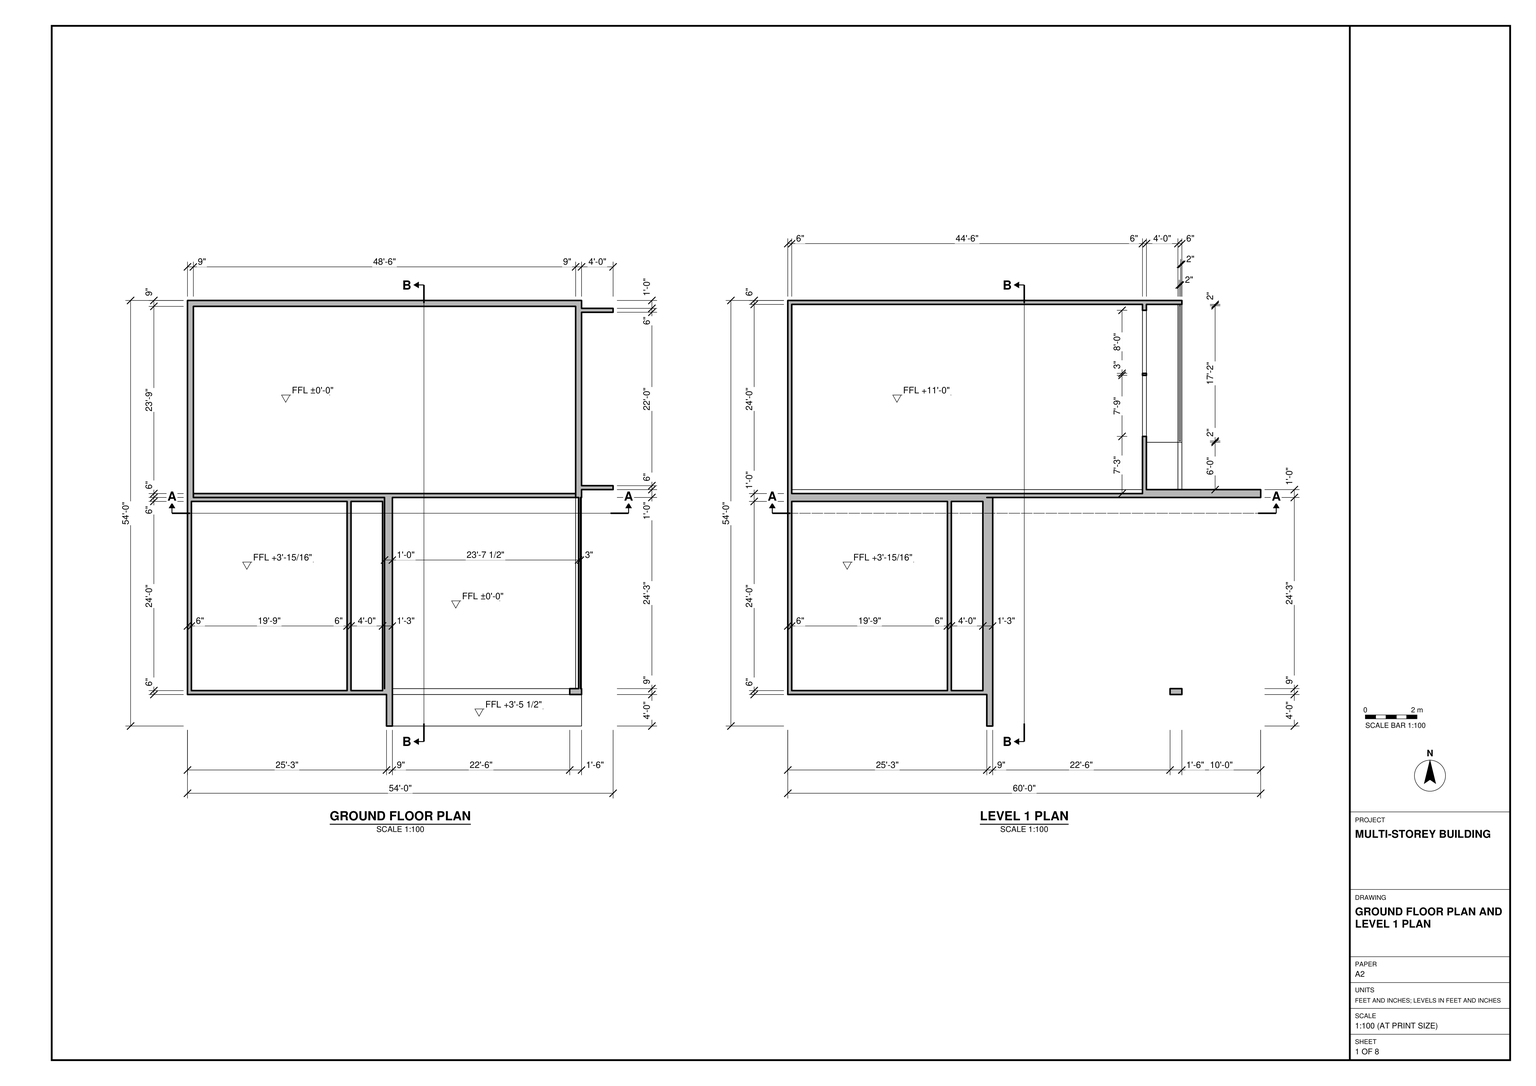
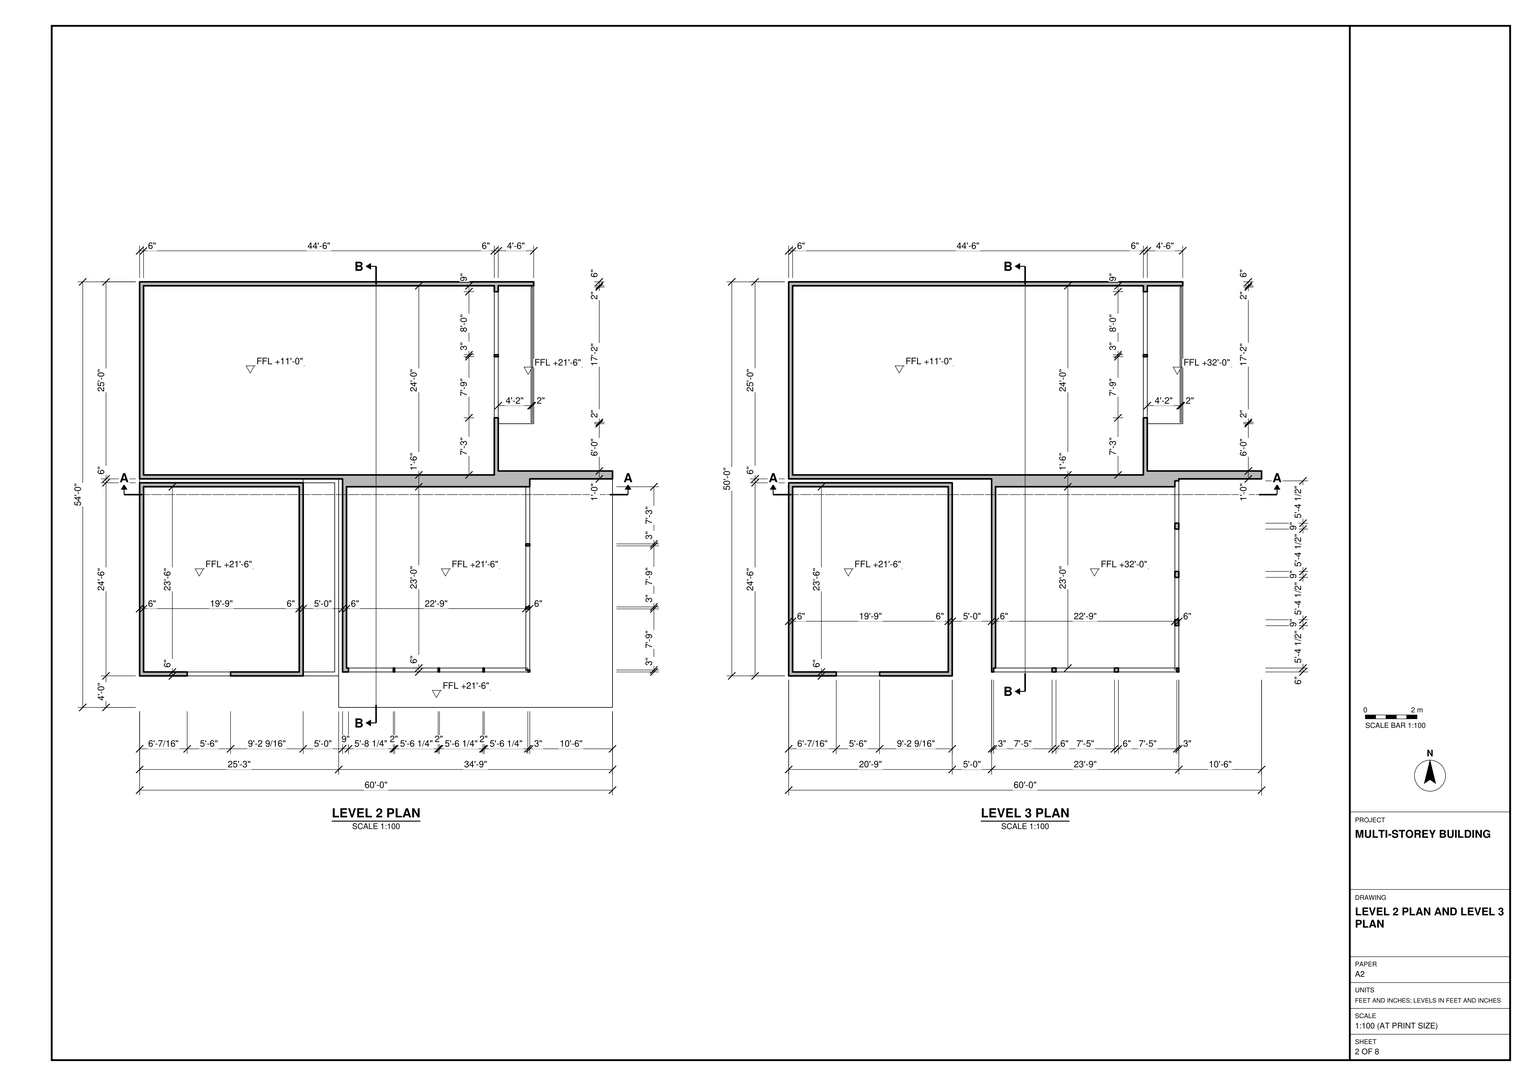
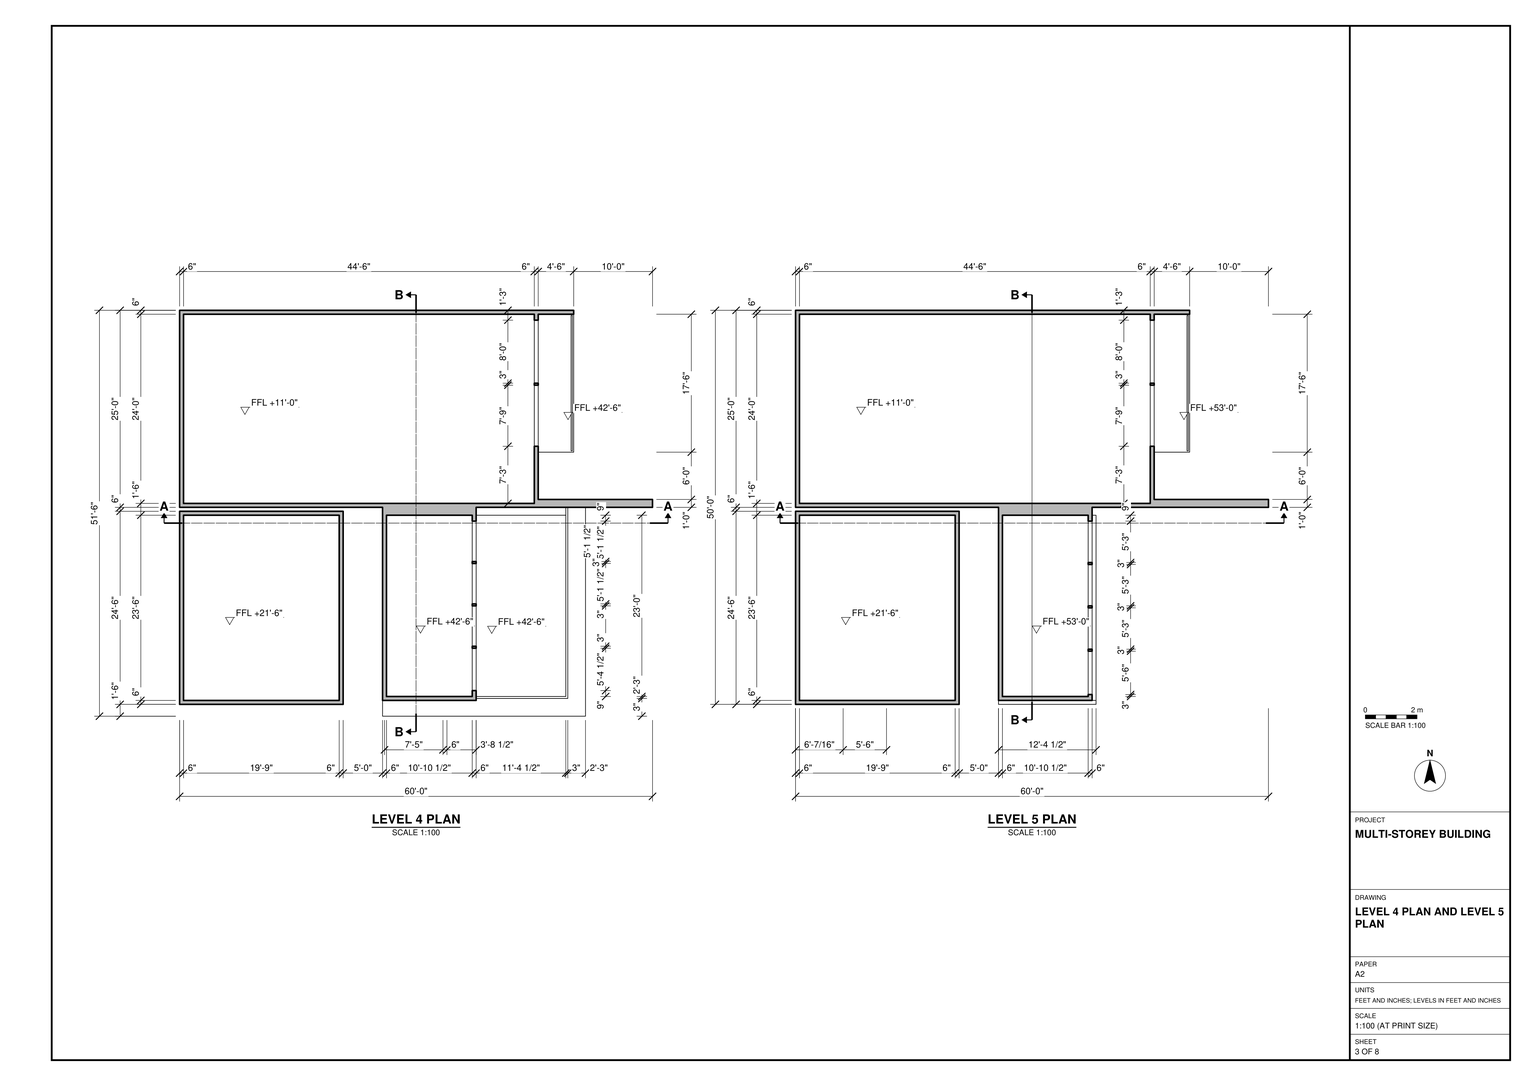
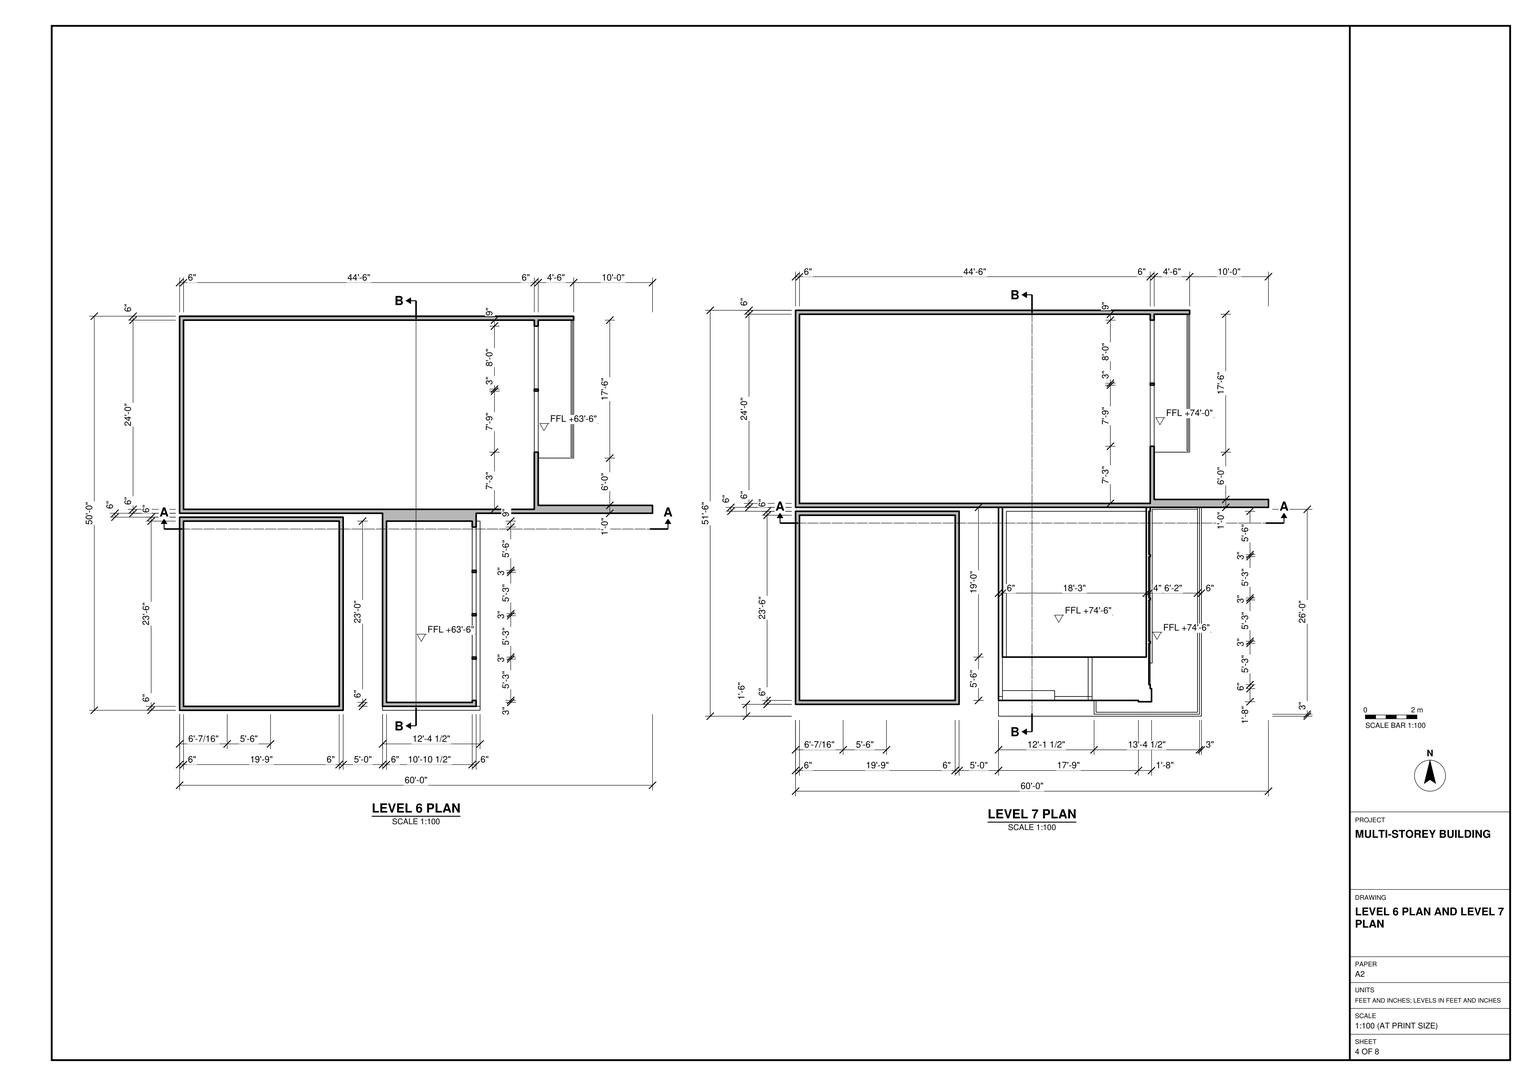
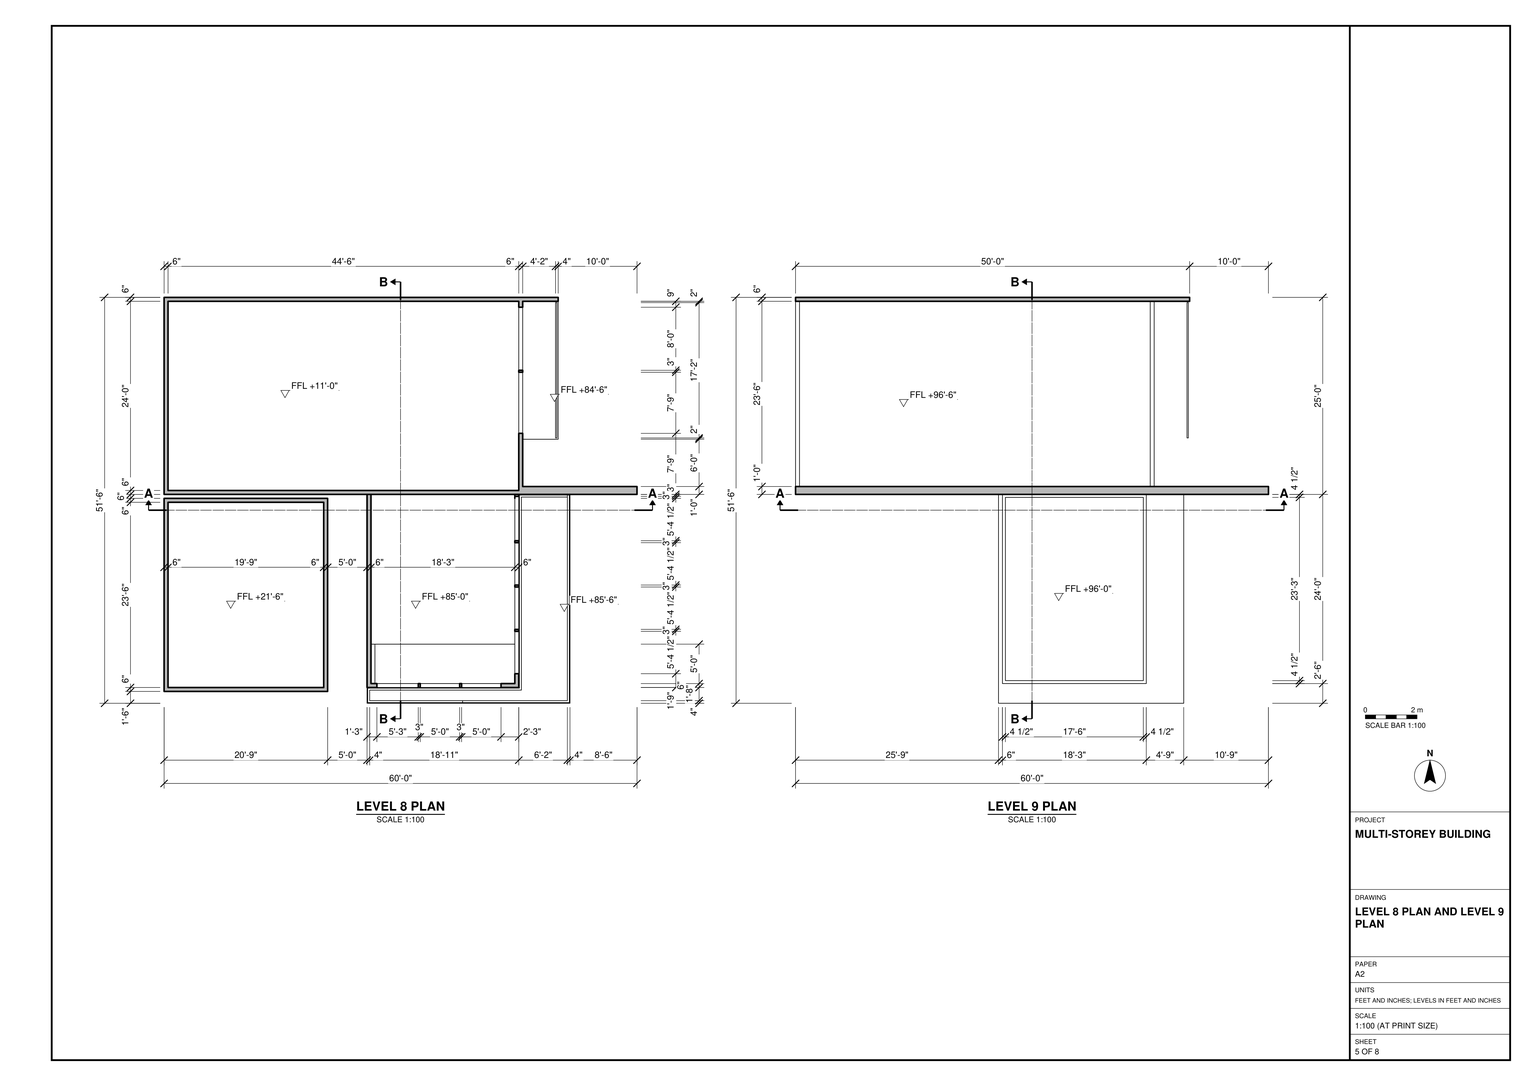
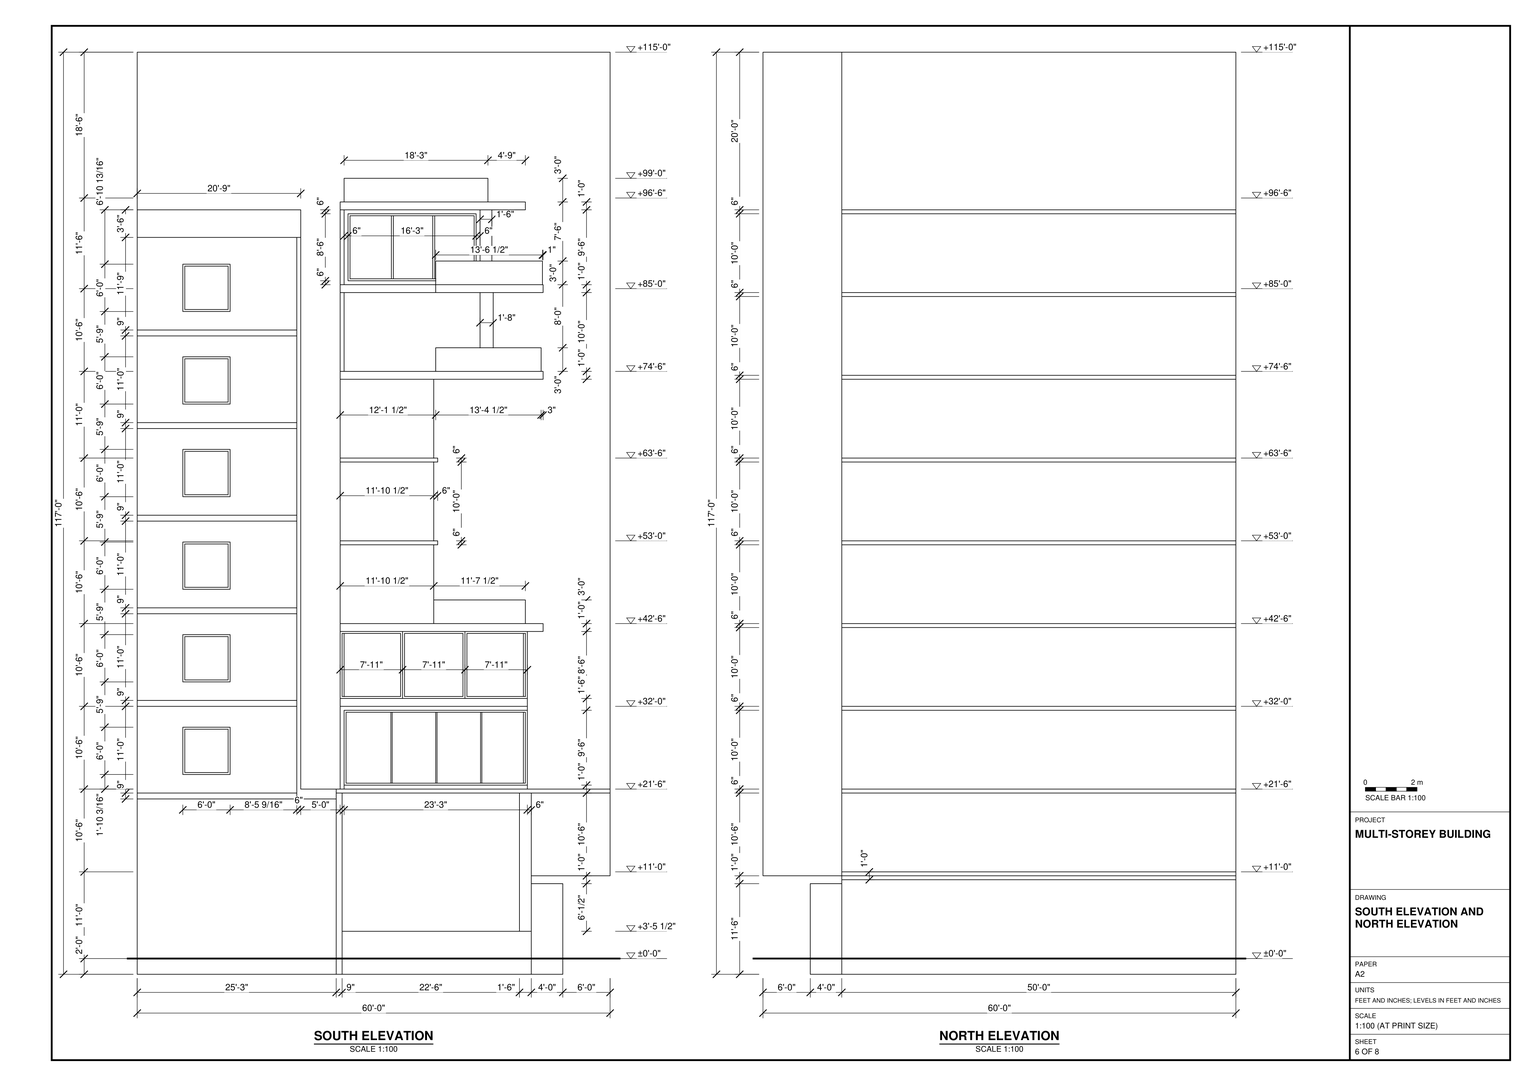
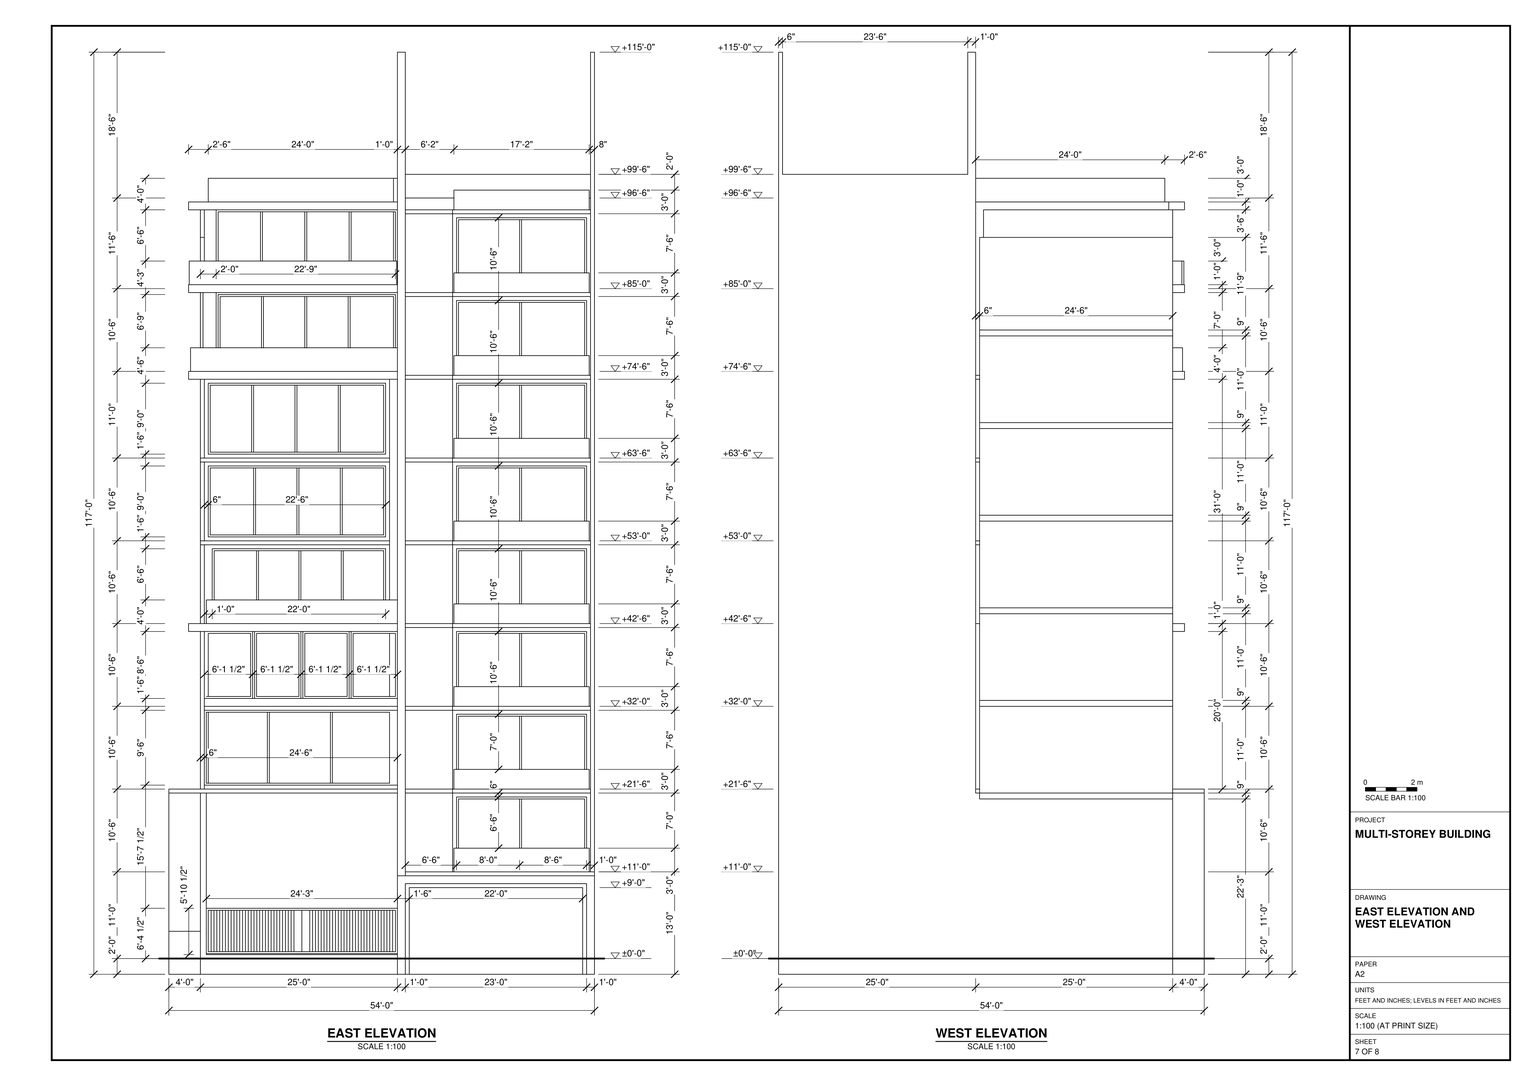
Build the multi-storey building in SketchUp from task_files/diagram_01.pdf. Work in feet and inches. The overall dimensions, including projections, are 60'-0" east to west, 54'-0" north to south and 117'-0" high. Use the storey levels ±0'-0", +11'-0", +21'-6", +32'-0", +42'-6", +53'-0", +63'-6", +74'-6", +85'-0" and +96'-6".

Start with the broad northern enclosure and the smaller bays to its south. Use the wall thicknesses shown for each bay rather than a single thickness throughout. Trace each floor slab separately: where a plan shows a floor at a lower level, leave the space above it open. Keep the gap between the southern bays, the narrowing of the southeastern enclosure and the slab edges that project beyond the walls. Place the openings and window units according to the plans, and use the sections to set their heights and complete the roof profile.

Keep walls, slabs and roof elements in separate groups or components. Keep each furniture or joinery piece shown separate as well, and use components for repeated parts. Any decor or loose items shown may be suitable library components. Save one SketchUp model as output_files/multi_storey_building_with_stepped_floor_plates.skp.

# SketchUp Ruby script. Lengths in inches.
U = 1.inch
M = Sketchup.active_model
def pt(a) = Geom::Point3d.new(a.map { |v| v * U })
def face(e, loops, mat)
  f = e.add_face(loops[0].map { |a| pt(a) })
  loops[1..].each { |l| e.add_face(l.map { |a| pt(a) }).erase! }
  f.material = f.back_material = mat if mat
  f
end
# faces: each face lists its corners as indices into pts; further lists are holes
def faces(e, pts, list, mat = nil) = list.each { |f| face(e, (f[0].is_a?(Array) ? f : [f]).map { |l| l.map { |i| pts[i] } }, mat) }
# xy, xz, yz: faces in a plane at the given z, y or x. An outline is a flat list of corners, or four numbers for a rectangle; further outlines are holes
def ring(l) = l.size == 4 ? [[l[0], l[1]], [l[2], l[1]], [l[2], l[3]], [l[0], l[3]]] : l.each_slice(2).to_a
def flat(e, list, mat, &to3) = list.each { |f| face(e, (f[0].is_a?(Array) ? f : [f]).map { |l| ring(l).map { |u, v| to3.(u, v) } }, mat) }
def xy(e, z, list, mat = nil) = flat(e, list, mat) { |x, y| [x, y, z] }
def xz(e, y, list, mat = nil) = flat(e, list, mat) { |x, z| [x, y, z] }
def yz(e, x, list, mat = nil) = flat(e, list, mat) { |y, z| [x, y, z] }
def lines(e, pts, list) = list.each { |a, b| e.add_line(pt(pts[a]), pt(pts[b])) }
# prism: a flat outline (further loops are holes) pulled along v
def prism(e, loops, v, mat = nil)
  f = face(e, loops, mat); d = Geom::Vector3d.new(v.map { |x| x * U })
  f.pushpull(f.normal.samedirection?(d) ? d.length : -d.length)
end
def box(e, o, s, mat = nil) = prism(e, [[o, [o[0] + s[0], o[1], o[2]], [o[0] + s[0], o[1] + s[1], o[2]], [o[0], o[1] + s[1], o[2]]]], [0, 0, s[2]], mat)
def at(x, y, z, deg = 0) = Geom::Transformation.translation(pt([x, y, z])) * Geom::Transformation.rotation(ORIGIN, Z_AXIS, deg.degrees)
def axes(o, x, y, z) = Geom::Transformation.new([*x, 0, *y, 0, *z, 0, *pt(o).to_a, 1])
def part(name) = M.definitions.add(name)
# library, detail: a bought-in or finely detailed component or shape, given as its bounding box
def library(name, o, s) = part(name).tap { |d| box(d.entities, o, s) }
def detail(e, o, s) = box(e.add_group.entities, o, s)
def put(e, d, t, mat = nil) = e.add_instance(d, t).tap { |i| i.material = mat if mat }
def group(e, t, mat = nil) = e.add_group.tap { |g| g.transformation = t; g.material = mat if mat }.entities
root = M.entities
M.materials.add("Glass_Basic_01").color = [161, 173, 186]
M.materials["Glass_Basic_01"].alpha = 0.25
M.materials.add("Plywood_01_1K").color = [125, 96, 64]
M.materials.add("ThomThom - Waistcoat1").color = [209, 209, 209]
M.materials.add("ThomThom - Waistcoat2").color = [127, 127, 126]
M.materials.add("Wood_Veneer_15_1K").color = [103, 69, 45]
c1 = part("Group\#2")
box(c1.entities,[0,0,0],[2,206,36])
g1 = group(root,at(0,48,0),"ThomThom - Waistcoat1")
xy(g1,0,[[303,-48,303,0,0,0,0,600,600,600,600,588,648,588,648,582,600,582,600,318,648,318,648,312,600,312,600,0,312,0,312,-48],[312,-48,600,0]])
xy(g1,24,[[9,9,300,300],[312,9,591,300],[9,306,591,591]])
xy(g1,30,[[312,0,582,9],[591,9,600,300]])
xy(g1,31.5,[[595.5,9,598.5,300]])
xy(g1,60.94,[[6,6,243,294],[249,6,297,294]])
xy(g1,65.48,[[312,-48,600,0]])
xy(g1,100.5,[[595.5,9,598.5,300]])
xy(g1,132,[[600,318,648,582]])
xy(g1,138,[[600,312,648,588]])
xy(g1,150,[[600,300,720,306],[9,306,591,591],[591,306,600,591],[600,306,720,312],[9,591,600,600]])
xy(g1,156,[[6,306,540,312],[6,312,540,594],[546,312,594,384],[594,312,600,384],[546,384,594,594],
  [594,384,600,594]])
xy(g1,165,[[540,393,546,486],[540,489,546,585]])
xy(g1,267,[[540,393,546,486],[540,489,546,585]])
xy(g1,276,[[303,-48,312,9],[312,-48,312,9,582,9,582,0,594,0,594,-48],[594,-48,720,0],[0,0,6,294],[6,0,243,6],
  [582,0,594,9],[594,0,600,9],[600,0,720,9],[6,6,243,294],[303,9,312,300],
  [312,9,591,300],[591,9,720,300],[0,294,249,300]])
xy(g1,276,[[546,384,600,594]],"Wood_Veneer_15_1K")
xy(g1,282,[[249,0,303,0,303,300,249,300,249,294,297,294,297,6,249,6],[6,6,243,288],[315,12,588,288],[546,384,600,594]])
xy(g1,282,[[303,-48,720,-48,720,300,594,300,594,6,309,6,309,300,303,300]],"Wood_Veneer_15_1K")
xy(g1,291,[[588,9,591,12],[540,393,546,486],[540,489,546,585]])
xy(g1,291,[[318,6,386.25,12],[388.25,6,454.5,12],[456.5,6,522.75,12],[524.75,6,591,6,591,9,588,9,588,12,524.75,12],[591,9,594,9,594,102,588,102,588,12,591,12],
  [588,105,594,198],[588,201,594,288]],"Wood_Veneer_15_1K")
xy(g1,307.22,[[72.45,0,138.45,6]])
xy(g1,373.22,[[72.45,0,138.45,6]])
xy(g1,393,[[540,393,546,486],[540,489,546,585]])
xy(g1,399,[[588,9,591,12]])
xy(g1,399,[[318,6,386.25,12],[388.25,6,454.5,12],[456.5,6,522.75,12],[524.75,6,524.75,12,588,12,588,9,591,9,591,6],[591,9,591,12,588,12,588,102,594,102,594,9],
  [588,105,594,198],[588,201,594,288]],"Wood_Veneer_15_1K")
xy(g1,402,[[315,12,588,288]])
xy(g1,402,[[546,384,600,594]],"Wood_Veneer_15_1K")
xy(g1,408,[[315,12,588,288],[546,384,600,594]])
xy(g1,417,[[540,393,546,486],[540,489,546,585]])
xy(g1,423,[[312,6,401,12],[407,6,496,12],[502,6,591,6,591,9,588,9,588,12,502,12],[588,9,591,12],[591,9,594,12],
  [588,12,594,76.5],[588,85.5,594,150],[588,159,594,223.5],[588,232.5,594,297]])
xy(g1,448.22,[[72.45,0,138.45,6]])
xy(g1,514.22,[[72.45,0,138.45,6]])
xy(g1,519,[[312,6,401,12],[407,6,496,12],[502,6,502,12,588,12,588,76.5,594,76.5,594,12,591,12,591,6],[588,85.5,594,150],[588,159,594,223.5],
  [588,232.5,594,297],[540,393,546,486],[540,489,546,585]])
xy(g1,522,[[309,-18,594,6],[594,-18,618,300]])
xy(g1,528,[[315,12,588,288]])
xy(g1,528,[[546,384,600,594]],"Wood_Veneer_15_1K")
xy(g1,534,[[309,-18,618,-18,618,300,591,300,591,9,451.5,9,451.5,6,309,6],[315,12,445.5,288],[451.5,12,588,288],[451.5,288,588,300],[546,384,600,594]])
xy(g1,543,[[445.5,21,451.5,85.5],[445.5,88.5,451.5,150],[445.5,153,451.5,214.5],[445.5,217.5,451.5,279],[540,393,546,486],
  [540,489,546,585]])
xy(g1,570,[[451.5,9,591,9,591,300,588,300,588,12,451.5,12]])
xy(g1,589.22,[[72.45,0,138.45,6]])
xy(g1,645,[[445.5,21,451.5,85.5],[445.5,88.5,451.5,150],[445.5,153,451.5,214.5],[445.5,217.5,451.5,279],[540,393,546,486],
  [540,489,546,585]])
xy(g1,654,[[309,0,457.5,6],[451.5,6,457.5,288],[315,12,445.5,288]])
xy(g1,654,[[546,384,600,594]],"Wood_Veneer_15_1K")
xy(g1,655.22,[[72.45,0,138.45,6]])
xy(g1,660,[[309,0,457.5,6],[451.5,6,457.5,288],[315,12,445.5,288],[546,384,600,594]])
xy(g1,669,[[445.5,15,451.5,81],[445.5,84,451.5,147],[445.5,150,451.5,213],[445.5,216,451.5,279],[540,393,546,486],
  [540,489,546,585]])
xy(g1,730.22,[[72.45,0,138.45,6]])
xy(g1,771,[[445.5,15,451.5,81],[445.5,84,451.5,147],[445.5,150,451.5,213],[445.5,216,451.5,279],[540,393,546,486],
  [540,489,546,585]])
xy(g1,780,[[309,0,457.5,6],[451.5,6,457.5,288],[315,12,445.5,288]])
xy(g1,780,[[546,384,600,594]],"Wood_Veneer_15_1K")
xy(g1,786,[[309,0,457.5,6],[451.5,6,457.5,288],[315,12,445.5,288],[546,384,600,594]])
xy(g1,795,[[445.5,15,451.5,78],[445.5,81,451.5,144],[445.5,147,451.5,210],[445.5,213,451.5,279],[540,393,546,486],
  [540,489,546,585]])
xy(g1,796.22,[[72.45,0,138.45,6]])
xy(g1,871.22,[[72.45,0,138.45,6]])
xy(g1,897,[[445.5,15,451.5,78],[445.5,81,451.5,144],[445.5,147,451.5,210],[445.5,213,451.5,279],[540,393,546,486],
  [540,489,546,585]])
xy(g1,906,[[309,-18,309,6,451.5,6,451.5,300,618,300,618,-18],[309,6,315,12],[315,6,445.5,12],[445.5,6,451.5,12],[309,12,315,300],
  [315,12,445.5,288],[445.5,12,451.5,300],[315,288,445.5,300]])
xy(g1,906,[[546,384,600,594]],"Wood_Veneer_15_1K")
xy(g1,912,[[546,384,600,594]])
xy(g1,918,[[309,-18,618,-18,618,300,615,300,615,-15,454.5,-15,454.5,6,309,6],[457.5,-12,612,-12,612,297,543,297,543,63,540,63,540,24,542,24,542,4,522,4,522,6,457.5,6],[315,6,394.5,21],[540,63,543,63,543,297,612,297,612,300,540,300],[315,72,321,72,321,294,534,294,534,300,315,300],
  [321,72,534,294]])
xy(g1,921,[[540,393,546,486],[540,489,546,585]])
xy(g1,924,[[538,30,540,63],[538,63,540,93],[538,96,540,159],[538,162,540,225],[538,228,540,294]])
xy(g1,937.22,[[72.45,0,138.45,6]])
xy(g1,954,[[454.5,-15,615,-15,615,300,612,300,612,-12,457.5,-12,457.5,6,454.5,6]])
xy(g1,1012.22,[[72.45,0,138.45,6]])
xy(g1,1023,[[540,393,546,486],[540,489,546,585]])
xy(g1,1032,[[538,30,540,66],[538,66,540,93],[538,96,540,159],[538,162,540,225],[538,228,540,294]])
xy(g1,1032,[[546,384,600,594]],"Wood_Veneer_15_1K")
xy(g1,1038,[[309,-18,457.5,6],[457.5,-18,457.5,6,522,6,522,4,542,4,542,24,540,24,540,66,618,66,618,-18],[540,66,618,300],[315,72,534,300],[546,384,600,594]])
xy(g1,1044,[[315,12,321,72],[321,12,534,72],[315,72,534,300]])
xy(g1,1047,[[540,393,546,486],[540,489,546,585]])
xy(g1,1050,[[309,-18,454.5,-18,454.5,-17,310,-17,310,5,541,5,541,299,617,299,617,-17,454.5,-17,454.5,-18,618,-18,618,300,540,300,540,6,309,6],[310,-17,454.5,-17,454.5,-14,313,-14,313,2,544,2,544,296,614,296,614,299,541,299,541,5,310,5],[313,-14,614,-14,614,296,544,296,544,2,313,2]])
xy(g1,1053,[[534,27,540,91.5],[534,94.5,540,159],[534,162,540,226.5],[534,229.5,540,297]])
xy(g1,1059,[[324,6,387,12],[390,6,450,12],[453,6,513,12]])
xy(g1,1078.22,[[72.45,0,138.45,6]])
xy(g1,1086,[[454.5,-17,617,-17,617,299,614,299,614,-14,454.5,-14]])
xy(g1,1122,[[0,0,6,288],[6,0,249,6],[6,6,243,288],[243,6,249,288],[0,288,249,294]])
xy(g1,1128,[[6,6,243,282]])
xy(g1,1149,[[540,393,546,486],[540,489,546,585]])
xy(g1,1155,[[324,6,387,12],[390,6,394.5,12],[394.5,6,450,12],[453,6,513,12]])
xy(g1,1158,[[546,384,600,594]],"Wood_Veneer_15_1K")
xy(g1,1161,[[534,27,540,91.5],[534,94.5,540,159],[534,162,540,226.5],[534,229.5,540,297]])
xy(g1,1164,[[309,-18,394.5,6],[394.5,-18,540,6],[540,-18,591,300],[[0,0,249,288],[6,6,243,282]],[315,12,534,300],
  [546,384,600,594]])
xy(g1,1176,[[309,-18,591,-18,591,300,534,300,534,12,315,12,315,300,309,300],[319.5,16.5,529.5,295.5],[6,306,540,594]])
xy(g1,1182,[[6,306,540,312],[6,312,540,594]])
xy(g1,1212,[[[315,12,534,300],[319.5,16.5,529.5,295.5]]])
xy(g1,1218,[[0,312,6,594],[540,312,546,594]])
xy(g1,1404,[[0,300,720,312],[0,594,600,600]])
xz(g1,-48,[[312,0,600,65.48]])
xz(g1,-48,[[303,0,312,276],[303,276,720,282]],"Wood_Veneer_15_1K")
xz(g1,-18,[[309,522,618,534],[309,906,618,918],[309,1038,454.5,1050],[454.5,1038,618,1050],[309,1164,591,1176]])
xz(g1,-17,[[454.5,1050,617,1086]],"Glass_Basic_01")
xz(g1,-15,[[454.5,918,615,954]],"Glass_Basic_01")
xz(g1,-14,[[454.5,1050,614,1086]],"Glass_Basic_01")
xz(g1,-12,[[457.5,918,612,954]],"Glass_Basic_01")
xz(g1,0,[[312,0,600,0,600,65.48,582,65.48,582,30,312,30],[312,30,582,65.48],[582,65.48,600,276],[0,267,243,276],[243,267,303,267,303,282,249,282,249,1122,243,1122],
  [[0,276,243,408],[69.45,304.22,141.45,376.22]],[[69.45,304.22,141.45,376.22],[72.45,307.22,138.45,373.22]],[0,408,243,417],[[0,417,243,549],[69.45,445.22,141.45,517.22]],[[69.45,445.22,141.45,517.22],[72.45,448.22,138.45,514.22]],
  [0,549,243,558],[[0,558,243,690],[69.45,586.22,141.45,658.22]],[[69.45,586.22,141.45,658.22],[72.45,589.22,138.45,655.22]],[309,654,457.5,660],[0,690,243,699],
  [[0,699,243,831],[69.45,727.22,141.45,799.22]],[[69.45,727.22,141.45,799.22],[72.45,730.22,138.45,796.22]],[309,780,457.5,786],[0,831,243,840],[[0,840,243,972],[69.45,868.22,141.45,940.22]],
  [[69.45,868.22,141.45,940.22],[72.45,871.22,138.45,937.22]],[0,972,243,981],[[0,981,243,1122],[69.45,1009.22,141.45,1081.22]],[[69.45,1009.22,141.45,1081.22],[72.45,1012.22,138.45,1078.22]],[0,1122,249,1164]])
xz(g1,0,[[0,0,303,267]],"ThomThom - Waistcoat2")
xz(g1,4,[[522,918,542,1038]],"ThomThom - Waistcoat1")
xz(g1,6,[[6,60.94,243,276],[249,60.94,297,282],[[6,282,243,1122],[72.45,871.22,138.45,937.22],[72.45,730.22,138.45,796.22],[72.45,589.22,138.45,655.22],[72.45,448.22,138.45,514.22],[72.45,307.22,138.45,373.22],[72.45,1012.22,138.45,1078.22]],[[309,420,404,522],[312,423,401,519]],[[404,420,499,522],[407,423,496,519]],
  [[499,420,594,522],[502,423,591,519]],[309,660,451.5,780],[309,786,451.5,906],[309,918,315,1038],[315,918,454.5,918,454.5,954,457.5,954,457.5,918,522,918,522,1038,315,1038],
  [309,1050,315,1164],[6,1128,243,1164]])
xz(g1,6,[[309,408,594,420],[522,1050,540,1164]],"ThomThom - Waistcoat1")
xz(g1,6,[[309,282,315,282,315,402,594,402,594,408,309,408],[315,282,594,288],[[315,288,594,402],[318,291,591,399]],[386.25,291,388.25,399],[454.5,291,456.5,399],
  [522.75,291,524.75,399],[309,534,451.5,654],[[315,1050,522,1164],[321,1056,516,1158]],[[321,1056,516,1158],[324,1059,513,1155]],[387,1059,390,1155],
  [450,1059,453,1155]],"Wood_Veneer_15_1K")
xz(g1,9,[[312,24,591,30],[[582,30,600,102],[595.5,31.5,598.5,100.5]],[582,102,582,276,594,276,594,150,600,150,600,102],[594,150,600,276],[588,291,594,399]])
xz(g1,9,[[451.5,534,591,570]],"Glass_Basic_01")
xz(g1,12,[[[315,282,315,402,588,402,588,399,524.75,399,524.75,291,588,291,588,282],[318,291,386.25,399],[456.5,291,522.75,399],[388.25,291,454.5,399]],[315,402,588,408],[[315,408,315,423,401,423,401,519,315,519,315,528,588,528,588,519,502,519,502,423,588,423,588,408],[407,423,496,519]],[312,423,315,519],[591,423,594,519],
  [315,534,445.5,654],[315,654,445.5,660],[315,660,445.5,780],[315,780,445.5,786],[315,786,445.5,906],
  [[315,1044,534,1164],[324,1059,387,1155],[453,1059,513,1155],[390,1059,450,1155]],[315,1164,534,1176]])
xz(g1,12,[[451.5,534,588,570],[315,1176,534,1212]],"Glass_Basic_01")
xz(g1,15,[[445.5,669,451.5,771],[445.5,795,451.5,897]])
xz(g1,16.5,[[319.5,1176,529.5,1212]],"Glass_Basic_01")
xz(g1,21,[[445.5,543,451.5,645]])
xz(g1,24,[[540,918,542,1038]],"ThomThom - Waistcoat1")
xz(g1,27,[[534,1053,540,1161]])
xz(g1,30,[[538,924,540,1032]])
xz(g1,72,[[315,918,321,1038],[321,918,534,1038],[315,1038,321,1044],[321,1038,534,1044]])
xz(g1,76.5,[[588,423,594,519]])
xz(g1,78,[[445.5,795,451.5,897]])
xz(g1,81,[[445.5,669,451.5,771],[445.5,795,451.5,897]])
xz(g1,84,[[445.5,669,451.5,771]])
xz(g1,85.5,[[588,423,594,519],[445.5,543,451.5,645]])
xz(g1,88.5,[[445.5,543,451.5,645]])
xz(g1,91.5,[[534,1053,540,1161]],"Wood_Veneer_15_1K")
xz(g1,93,[[538,924,540,1032]])
xz(g1,94.5,[[534,1053,540,1161]])
xz(g1,96,[[538,924,540,1032]])
xz(g1,102,[[588,291,594,399]],"Wood_Veneer_15_1K")
xz(g1,105,[[588,291,594,399]])
xz(g1,144,[[445.5,795,451.5,897]])
xz(g1,147,[[445.5,669,451.5,771],[445.5,795,451.5,897]])
xz(g1,150,[[588,423,594,519],[445.5,543,451.5,645],[445.5,669,451.5,771]])
xz(g1,153,[[445.5,543,451.5,645]])
xz(g1,159,[[588,423,594,519],[538,924,540,1032]])
xz(g1,159,[[534,1053,540,1161]],"Wood_Veneer_15_1K")
xz(g1,162,[[538,924,540,1032],[534,1053,540,1161]])
xz(g1,198,[[588,291,594,399]],"Wood_Veneer_15_1K")
xz(g1,201,[[588,291,594,399]])
xz(g1,210,[[445.5,795,451.5,897]])
xz(g1,213,[[445.5,669,451.5,771],[445.5,795,451.5,897]])
xz(g1,214.5,[[445.5,543,451.5,645]])
xz(g1,216,[[445.5,669,451.5,771]])
xz(g1,217.5,[[445.5,543,451.5,645]])
xz(g1,223.5,[[588,423,594,519]])
xz(g1,225,[[538,924,540,1032]])
xz(g1,226.5,[[534,1053,540,1161]],"Wood_Veneer_15_1K")
xz(g1,228,[[538,924,540,1032]])
xz(g1,229.5,[[534,1053,540,1161]])
xz(g1,232.5,[[588,423,594,519]])
xz(g1,279,[[445.5,543,451.5,645],[445.5,669,451.5,771],[445.5,795,451.5,897]])
xz(g1,282,[[6,1128,243,1164]])
xz(g1,288,[[6,282,243,1122],[315,282,588,402],[315,402,588,408],[315,408,588,528],[315,534,445.5,654],
  [315,654,445.5,660],[451.5,654,457.5,660],[315,660,445.5,780],[315,780,445.5,786],[451.5,780,457.5,786],
  [315,786,445.5,906],[0,1122,249,1164]])
xz(g1,288,[[588,291,594,399]],"Wood_Veneer_15_1K")
xz(g1,294,[[6,60.94,243,276],[249,60.94,297,282],[0,276,243,1122],[243,276,249,1122],[538,924,540,1032]])
xz(g1,295.5,[[319.5,1176,529.5,1212]],"Glass_Basic_01")
xz(g1,297,[[588,423,594,519]])
xz(g1,297,[[534,1053,540,1161]],"Wood_Veneer_15_1K")
xz(g1,299,[[614,1050,617,1086]])
xz(g1,300,[[9,24,300,150],[312,24,591,276],[[591,30,600,30,600,150,720,150,720,276,591,276],[595.5,31.5,598.5,100.5]],[303,156,306,276],[306,156,312,270],
  [306,270,312,276],[303,276,306,282],[306,276,312,282],[312,276,591,282],[591,276,720,282],
  [309,906,309,1176,315,1176,315,918,534,918,534,1176,591,1176,591,1164,540,1164,540,1050,618,1050,618,1038,540,1038,540,918,591,918,591,906],[591,906,591,918,612,918,612,954,615,954,615,918,618,918,618,906],[315,918,534,1038],[315,1038,534,1044],[315,1044,534,1164],
  [315,1164,534,1212]])
xz(g1,300,[[0,276,249,276,249,282,309,282,309,1176,315,1176,315,1212,534,1212,534,1176,591,1176,591,1164,540,1164,540,1050,618,1050,618,1038,540,1038,540,918,612,918,612,954,615,954,615,918,618,918,618,906,451.5,906,451.5,534,588,534,588,570,591,570,591,534,618,534,618,522,594,522,594,282,720,282,720,1404,0,1404]],"ThomThom - Waistcoat1")
xz(g1,306,[[9,24,591,150],[6,156,540,1176],[6,1176,540,1182]])
xz(g1,312,[[600,0,648,138]])
xz(g1,312,[[600,150,600,156,546,156,546,1218,540,1218,540,1182,6,1182,6,1218,0,1218,0,1404,720,1404,720,150]],"ThomThom - Waistcoat1")
xz(g1,318,[[600,0,648,132]])
xz(g1,384,[[546,276,600,282],[546,402,600,408],[546,528,600,534],[546,654,600,660],[546,780,600,786],
  [546,906,600,912],[546,1032,600,1038],[546,1158,600,1164]])
xz(g1,393,[[540,165,546,267],[540,291,546,393],[540,417,546,519],[540,543,546,645],[540,669,546,771],
  [540,795,546,897],[540,921,546,1023],[540,1047,546,1149]])
xz(g1,486,[[540,165,546,267],[540,291,546,393],[540,417,546,519],[540,543,546,645],[540,669,546,771],
  [540,795,546,897],[540,921,546,1023],[540,1047,546,1149]])
xz(g1,489,[[540,165,546,267],[540,291,546,393],[540,417,546,519],[540,543,546,645],[540,669,546,771],
  [540,795,546,897],[540,921,546,1023],[540,1047,546,1149]])
xz(g1,582,[[600,0,648,132]])
xz(g1,585,[[540,165,546,267],[540,291,546,393],[540,417,546,519],[540,543,546,645],[540,669,546,771],
  [540,795,546,897],[540,921,546,1023],[540,1047,546,1149]])
xz(g1,588,[[600,0,648,138]])
xz(g1,591,[[9,24,591,144],[9,144,591,150]])
xz(g1,594,[[6,156,540,1176],[546,156,600,276],[546,282,600,402],[546,408,600,528],[546,534,600,654],
  [546,660,600,780],[546,786,600,906],[546,912,600,1032],[546,1038,600,1158],[6,1176,540,1182],
  [0,1218,6,1404],[540,1218,546,1404]])
xz(g1,594,[[546,1164,600,1404],[6,1182,540,1404]],"ThomThom - Waistcoat1")
xz(g1,600,[[0,0,600,144],[0,144,600,150],[0,150,600,156],[0,156,600,276],[0,276,600,282],
  [0,282,600,402],[0,402,600,408],[0,408,600,528],[0,528,600,534],[0,534,600,654],
  [0,654,600,660],[0,660,600,780],[0,780,600,786],[0,786,600,906],[0,906,600,912],
  [0,912,600,1032],[0,1032,600,1038],[0,1038,600,1158],[0,1158,600,1164]])
xz(g1,600,[[0,1164,600,1404]],"ThomThom - Waistcoat1")
yz(g1,0,[[0,0,0,267,294,267,294,276,300,276,300,1404,312,1404,312,1218,594,1218,594,1404,600,1404,600,0],[0,267,294,276],[0,276,294,408],[0,408,294,417],[0,417,294,549],
  [0,549,294,558],[0,558,294,690],[0,690,294,699],[0,699,294,831],[0,831,294,840],
  [0,840,294,972],[0,972,294,981],[0,981,294,1122],[0,1122,288,1164]])
yz(g1,6,[[6,60.94,294,276],[306,156,312,1176],[312,156,594,1176],[6,282,288,1122],[6,1128,282,1164],
  [306,1176,312,1182],[312,1176,594,1182],[312,1182,594,1218]])
yz(g1,9,[[300,24,306,144],[306,24,591,144],[300,144,306,150],[306,144,591,150]])
yz(g1,72.45,[[0,307.22,6,373.22],[0,448.22,6,514.22],[0,589.22,6,655.22],[0,730.22,6,796.22],[0,871.22,6,937.22],
  [0,1012.22,6,1078.22]])
yz(g1,138.45,[[0,307.22,6,373.22],[0,448.22,6,514.22],[0,589.22,6,655.22],[0,730.22,6,796.22],[0,871.22,6,937.22],
  [0,1012.22,6,1078.22]])
yz(g1,243,[[6,60.94,294,276],[6,282,288,1122],[6,1128,282,1164]])
yz(g1,249,[[6,60.94,294,282],[294,276,300,282],[0,282,6,1122],[6,282,294,1122],[0,1122,288,1164]])
yz(g1,297,[[6,60.94,294,282]])
yz(g1,300,[[9,24,300,150]])
yz(g1,303,[[0,276,9,282],[9,276,300,282]])
yz(g1,303,[[-48,0,0,276],[-48,276,0,282]],"Wood_Veneer_15_1K")
yz(g1,309,[[6,282,300,534],[-18,522,6,534],[6,534,300,654],[0,654,300,660],[6,660,300,780],
  [0,780,300,786],[6,786,300,906],[-18,906,6,918],[6,906,6,1176,300,1176,300,912,12,912,12,906],[12,906,300,912],
  [-18,1038,6,1050],[-18,1164,6,1176]])
yz(g1,312,[[-48,0,0,65.48],[9,24,300,24,300,276,-48,276,-48,65.48,0,65.48,0,30,9,30],[6,423,12,519]])
yz(g1,315,[[12,282,288,402],[12,402,288,408],[12,408,288,528],[12,528,288,534],[12,534,288,654],
  [12,654,288,660],[12,660,288,780],[12,780,288,786],[12,786,288,906],[72,918,300,1038],
  [72,1038,300,1044],[12,1044,300,1164],[12,1164,300,1176]])
yz(g1,315,[[12,1176,300,1212]],"Glass_Basic_01")
yz(g1,318,[[6,291,12,399]],"Wood_Veneer_15_1K")
yz(g1,319.5,[[16.5,1176,295.5,1212]],"Glass_Basic_01")
yz(g1,324,[[6,1059,12,1155]],"Wood_Veneer_15_1K")
yz(g1,386.25,[[6,291,12,399]])
yz(g1,387,[[6,1059,12,1155]])
yz(g1,388.25,[[6,291,12,399]],"Wood_Veneer_15_1K")
yz(g1,390,[[6,1059,12,1155]],"Wood_Veneer_15_1K")
yz(g1,401,[[6,423,12,519]])
yz(g1,407,[[6,423,12,519]])
yz(g1,445.5,[[[12,534,288,654],[21,543,85.5,645],[217.5,543,279,645],[88.5,543,150,645],[153,543,214.5,645]],[12,654,288,660],[[12,660,288,780],[15,669,81,771],[150,669,213,771],[216,669,279,771],[84,669,147,771]],[12,780,288,786],[[12,786,288,906],[213,795,279,897],[147,795,210,897],[15,795,78,897],[81,795,144,897]]])
yz(g1,450,[[6,1059,12,1155]])
yz(g1,451.5,[[[6,534,9,534,9,570,12,570,12,534,288,534,288,654,6,654],[18,540,282,648]],[288,534,300,906],[[18,540,282,648],[21,543,279,645]],[85.5,543,88.5,645],[150,543,153,645],
  [214.5,543,217.5,645],[[6,660,288,780],[12,666,282,774]],[[12,666,282,774],[15,669,279,771]],[81,669,84,771],[147,669,150,771],
  [213,669,216,771],[[6,786,288,906],[12,792,282,900]],[[12,792,282,900],[15,795,279,897]],[78,795,81,897],[144,795,147,897],
  [210,795,213,897]],"Wood_Veneer_15_1K")
yz(g1,453,[[6,1059,12,1155]],"Wood_Veneer_15_1K")
yz(g1,454.5,[[6,291,12,399],[-17,1050,-14,1086]])
yz(g1,454.5,[[-15,918,6,954]],"Glass_Basic_01")
yz(g1,456.5,[[6,291,12,399]],"Wood_Veneer_15_1K")
yz(g1,457.5,[[0,654,288,660],[0,780,288,786]])
yz(g1,457.5,[[-12,918,6,954]],"Glass_Basic_01")
yz(g1,496,[[6,423,12,519]])
yz(g1,502,[[6,423,12,519]])
yz(g1,513,[[6,1059,12,1155]])
yz(g1,522,[[4,918,6,1038]],"ThomThom - Waistcoat1")
yz(g1,522.75,[[6,291,12,399]])
yz(g1,524.75,[[6,291,12,399]],"Wood_Veneer_15_1K")
yz(g1,529.5,[[294,1176,295.5,1212]])
yz(g1,529.5,[[16.5,1176,294,1212]],"Glass_Basic_01")
yz(g1,534,[[72,918,294,1038],[294,918,300,1038],[72,1038,294,1044],[294,1038,300,1044],[[12,1044,12,1164,294,1164,294,1161,229.5,1161,229.5,1053,294,1053,294,1044],[162,1053,226.5,1161],[27,1053,91.5,1161],[94.5,1053,159,1161]],
  [294,1044,294,1053,297,1053,297,1161,294,1161,294,1164,300,1164,300,1044],[294,1053,297,1161],[12,1164,294,1176],[294,1164,300,1176],[294,1176,300,1212]])
yz(g1,534,[[12,1176,294,1212]],"Glass_Basic_01")
yz(g1,538,[[30,924,93,1032],[96,924,159,1032],[162,924,225,1032],[228,924,294,1032]])
yz(g1,540,[[306,156,312,1176],[[312,156,594,1176],[489,165,585,267],[489,291,585,393],[489,417,585,519],[489,543,585,645],[489,669,585,771],[489,795,585,897],[489,921,585,1023],[489,1047,585,1149],[393,165,486,267],[393,291,486,393],[393,417,486,519],[393,543,486,645],[393,669,486,771],[393,795,486,897],[393,921,486,1023],[393,1047,486,1149]],[306,1176,312,1182],[312,1176,594,1182]])
yz(g1,540,[[312,1182,594,1218]],"Glass_Basic_01")
yz(g1,540,[[6,1050,24,1164]],"ThomThom - Waistcoat1")
yz(g1,540,[[[24,918,300,1038],[27,921,297,1035]],[[27,921,297,1035],[30,924,294,1032]],[93,924,96,1032],[159,924,162,1032],[225,924,228,1032],
  [[24,1050,300,1164],[27,1053,297,1161]],[91.5,1053,94.5,1161],[159,1053,162,1161],[226.5,1053,229.5,1161]],"Wood_Veneer_15_1K")
yz(g1,542,[[4,918,24,1038]],"ThomThom - Waistcoat1")
yz(g1,546,[[[384,156,594,276],[390,162,588,270]],[312,276,384,282],[[384,282,594,402],[390,288,588,396]],[312,402,384,408],[[384,408,594,528],[390,414,588,522]],
  [312,528,384,534],[[384,534,594,654],[390,540,588,648]],[312,654,384,660],[[384,660,594,780],[390,666,588,774]],[312,780,384,786],
  [[384,786,594,906],[390,792,588,900]],[312,906,384,912],[[384,912,594,1032],[390,918,588,1026]],[312,1032,384,1038],[[384,1038,594,1158],[390,1044,588,1152]],
  [312,1158,384,1164],[312,1164,594,1182]])
yz(g1,546,[[312,1182,594,1218]],"Glass_Basic_01")
yz(g1,546,[[312,156,384,276],[[390,162,588,270],[393,165,585,267]],[486,165,489,267],[312,282,384,402],[[390,288,588,396],[393,291,585,393]],
  [486,291,489,393],[312,408,384,528],[[390,414,588,522],[393,417,585,519]],[486,417,489,519],[312,534,384,654],
  [[390,540,588,648],[393,543,585,645]],[486,543,489,645],[312,660,384,780],[[390,666,588,774],[393,669,585,771]],[486,669,489,771],
  [312,786,384,906],[[390,792,588,900],[393,795,585,897]],[486,795,489,897],[312,912,384,1032],[[390,918,588,1026],[393,921,585,1023]],
  [486,921,489,1023],[312,1038,384,1158],[[390,1044,588,1152],[393,1047,585,1149]],[486,1047,489,1149]],"Wood_Veneer_15_1K")
yz(g1,582,[[0,30,9,276]])
yz(g1,588,[[[12,282,12,291,102,291,102,399,12,399,12,402,288,402,288,399,201,399,201,291,288,291,288,282],[105,291,198,399]],[12,402,288,408],[[12,408,12,423,76.5,423,76.5,519,12,519,12,528,288,528,288,519,232.5,519,232.5,423,288,423,288,408],[85.5,423,150,519],[159,423,223.5,519]],[288,423,297,519],[12,528,288,534],
  [288,534,300,570]])
yz(g1,588,[[12,534,288,570]],"Glass_Basic_01")
yz(g1,591,[[9,24,294,30],[294,24,300,30],[300,24,306,144],[306,24,591,144],[300,144,306,150],
  [306,144,591,150],[6,423,12,519],[-18,1164,300,1176]])
yz(g1,591,[[9,534,300,570]],"Glass_Basic_01")
yz(g1,594,[[6,408,300,420]],"ThomThom - Waistcoat1")
yz(g1,594,[[6,282,300,288],[[6,288,300,402],[9,291,288,399]],[102,291,105,399],[198,291,201,399],[6,402,300,408],
  [[6,420,79.5,522],[12,423,76.5,519]],[79.5,420,82.5,522],[[82.5,420,153,522],[85.5,423,150,519]],[153,420,156,522],[[156,420,226.5,522],[159,423,223.5,519]],
  [226.5,420,229.5,522],[[229.5,420,300,522],[232.5,423,297,519]]],"Wood_Veneer_15_1K")
yz(g1,595.5,[[9,31.5,300,100.5]])
yz(g1,598.5,[[142.5,34.5,154.5,97.5],[154.5,34.5,166.5,97.5]],"Plywood_01_1K")
yz(g1,598.5,[[[9,31.5,300,100.5],[12,34.5,297,97.5]],[12,34.5,16.35,97.5],[16.35,34.5,20.7,97.5],[20.7,34.5,25.05,97.5],[25.05,34.5,29.4,97.5],
  [29.4,34.5,33.75,97.5],[33.75,34.5,38.1,97.5],[38.1,34.5,42.45,97.5],[42.45,34.5,46.8,97.5],[46.8,34.5,51.15,97.5],
  [51.15,34.5,55.5,97.5],[55.5,34.5,59.85,97.5],[59.85,34.5,64.2,97.5],[64.2,34.5,68.55,97.5],[68.55,34.5,72.9,97.5],
  [72.9,34.5,77.25,97.5],[77.25,34.5,81.6,97.5],[81.6,34.5,85.95,97.5],[85.95,34.5,90.3,97.5],[90.3,34.5,94.65,97.5],
  [94.65,34.5,99,97.5],[99,34.5,103.35,97.5],[103.35,34.5,107.7,97.5],[107.7,34.5,112.05,97.5],[112.05,34.5,116.4,97.5],
  [116.4,34.5,120.75,97.5],[120.75,34.5,125.1,97.5],[125.1,34.5,129.45,97.5],[129.45,34.5,133.8,97.5],[133.8,34.5,138.15,97.5],
  [138.15,34.5,142.5,97.5],[166.5,34.5,170.85,97.5],[170.85,34.5,175.2,97.5],[175.2,34.5,179.55,97.5],[179.55,34.5,183.9,97.5],
  [183.9,34.5,188.25,97.5],[188.25,34.5,192.6,97.5],[192.6,34.5,196.95,97.5],[196.95,34.5,201.3,97.5],[201.3,34.5,205.65,97.5],
  [205.65,34.5,210,97.5],[210,34.5,214.35,97.5],[214.35,34.5,218.7,97.5],[218.7,34.5,223.05,97.5],[223.05,34.5,227.4,97.5],
  [227.4,34.5,231.75,97.5],[231.75,34.5,236.1,97.5],[236.1,34.5,240.45,97.5],[240.45,34.5,244.8,97.5],[244.8,34.5,249.15,97.5],
  [249.15,34.5,253.5,97.5],[253.5,34.5,257.85,97.5],[257.85,34.5,262.2,97.5],[262.2,34.5,266.55,97.5],[266.55,34.5,270.9,97.5],
  [270.9,34.5,275.25,97.5],[275.25,34.5,279.6,97.5],[279.6,34.5,283.95,97.5],[283.95,34.5,288.3,97.5],[288.3,34.5,292.65,97.5],
  [292.65,34.5,297,97.5]],"Wood_Veneer_15_1K")
yz(g1,600,[[-48,0,0,65.48],[0,0,300,0,300,30,9,30,9,276,0,276],[300,0,312,0,312,138,588,138,588,0,600,0,600,150,300,150],[318,0,582,132],[312,150,600,156],
  [594,156,600,1404],[384,276,594,282],[384,402,594,408],[384,528,594,534],[384,654,594,660],
  [384,780,594,786],[384,906,594,912],[384,1032,594,1038],[384,1158,594,1164]])
yz(g1,612,[[297,918,300,954]])
yz(g1,612,[[-12,918,297,954]],"Glass_Basic_01")
yz(g1,614,[[296,1050,299,1086]])
yz(g1,614,[[-14,1050,296,1086]],"Glass_Basic_01")
yz(g1,615,[[-15,918,300,954]],"Glass_Basic_01")
yz(g1,617,[[-17,1050,299,1086]],"Glass_Basic_01")
yz(g1,618,[[-18,522,300,534],[-18,906,300,918],[-18,1038,300,1050]])
yz(g1,648,[[312,0,318,0,318,132,582,132,582,0,588,0,588,138,312,138]])
yz(g1,720,[[300,150,312,1404],[-48,276,300,282]])
# 12 loose lines left out
put(g1,c1,at(596,386,156),"Glass_Basic_01")
put(g1,c1,at(596,386,276),"Glass_Basic_01")
put(g1,c1,at(596,386,402),"Glass_Basic_01")
put(g1,c1,at(596,386,528),"Glass_Basic_01")
put(g1,c1,at(596,386,654),"Glass_Basic_01")
put(g1,c1,at(596,386,780),"Glass_Basic_01")
put(g1,c1,at(596,386,906),"Glass_Basic_01")
put(g1,c1,at(596,386,1032),"Glass_Basic_01")
put(g1,c1,at(596,386,1158),"Glass_Basic_01")
